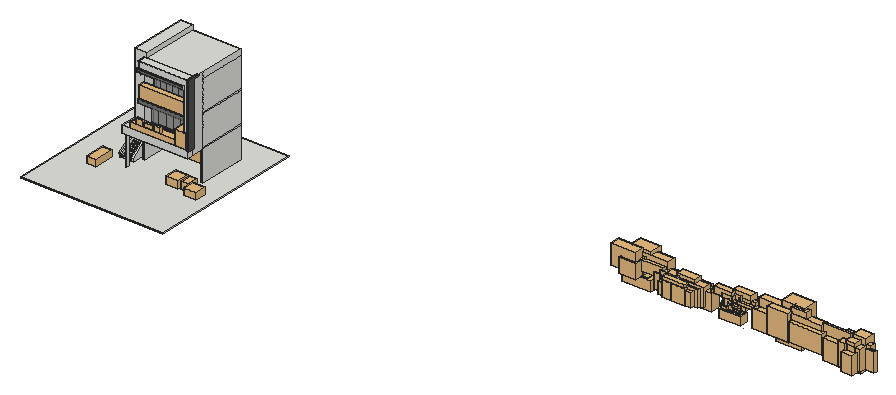
# SketchUp Ruby script. Lengths in inches.
U = 1.inch
M = Sketchup.active_model
def pt(a) = Geom::Point3d.new(a.map { |v| v * U })
def face(e, loops, mat)
  f = e.add_face(loops[0].map { |a| pt(a) })
  loops[1..].each { |l| e.add_face(l.map { |a| pt(a) }).erase! }
  f.material = f.back_material = mat if mat
  f
end
# faces: each face lists its corners as indices into pts; further lists are holes
def faces(e, pts, list, mat = nil) = list.each { |f| face(e, (f[0].is_a?(Array) ? f : [f]).map { |l| l.map { |i| pts[i] } }, mat) }
# xy, xz, yz: faces in a plane at the given z, y or x. An outline is a flat list of corners, or four numbers for a rectangle; further outlines are holes
def ring(l) = l.size == 4 ? [[l[0], l[1]], [l[2], l[1]], [l[2], l[3]], [l[0], l[3]]] : l.each_slice(2).to_a
def flat(e, list, mat, &to3) = list.each { |f| face(e, (f[0].is_a?(Array) ? f : [f]).map { |l| ring(l).map { |u, v| to3.(u, v) } }, mat) }
def xy(e, z, list, mat = nil) = flat(e, list, mat) { |x, y| [x, y, z] }
def xz(e, y, list, mat = nil) = flat(e, list, mat) { |x, z| [x, y, z] }
def yz(e, x, list, mat = nil) = flat(e, list, mat) { |y, z| [x, y, z] }
def lines(e, pts, list) = list.each { |a, b| e.add_line(pt(pts[a]), pt(pts[b])) }
# prism: a flat outline (further loops are holes) pulled along v
def prism(e, loops, v, mat = nil)
  f = face(e, loops, mat); d = Geom::Vector3d.new(v.map { |x| x * U })
  f.pushpull(f.normal.samedirection?(d) ? d.length : -d.length)
end
def box(e, o, s, mat = nil) = prism(e, [[o, [o[0] + s[0], o[1], o[2]], [o[0] + s[0], o[1] + s[1], o[2]], [o[0], o[1] + s[1], o[2]]]], [0, 0, s[2]], mat)
def at(x, y, z, deg = 0) = Geom::Transformation.translation(pt([x, y, z])) * Geom::Transformation.rotation(ORIGIN, Z_AXIS, deg.degrees)
def axes(o, x, y, z) = Geom::Transformation.new([*x, 0, *y, 0, *z, 0, *pt(o).to_a, 1])
def part(name) = M.definitions.add(name)
# library, detail: a bought-in or finely detailed component or shape, given as its bounding box
def library(name, o, s) = part(name).tap { |d| box(d.entities, o, s) }
def detail(e, o, s) = box(e.add_group.entities, o, s)
def put(e, d, t, mat = nil) = e.add_instance(d, t).tap { |i| i.material = mat if mat }
def group(e, t, mat = nil) = e.add_group.tap { |g| g.transformation = t; g.material = mat if mat }.entities
root = M.entities
M.materials.add("BANANA_BIG_STVOL_1").color = [93, 83, 53]
M.materials.add("POT_TEXTURE_1").color = [172, 172, 172]
M.materials.add("POT_TEXTURE_2").color = [160, 154, 144]
M.materials.add("[0135_DarkGray]").color = [81, 81, 81]
M.materials.add("[Color D06]").color = [204, 153, 0]
M.materials.add("[Metal Seamed]").color = [118, 119, 115]
M.materials.add("[Translucent Glass Sky Reflection]").color = [126, 138, 183]
M.materials["[Translucent Glass Sky Reflection]"].alpha = 0.52
M.materials.add("[Translucent_Glass_Gray]").color = [128, 128, 128]
M.materials["[Translucent_Glass_Gray]"].alpha = 0.5
M.materials.add("[Wood Square Tile 01]").color = [164, 91, 44]
M.materials.add("soil1").color = [68, 55, 47]
M.materials.add("white_concrete_pot1").color = [212, 211, 204]
M.materials.add("wood_1").color = [140, 119, 94]
c1 = library("sliding+glass+door+with+curtain",[16.58,6.29,0],[12.8,171.26,109.24])
c2 = part("Group\#3")
prism(c2.entities,[[[0,0,-94.49],[0,0,23.62],[-248.03,0,23.62],[-248.03,0,0],[-15.75,0,0],[-15.75,0,-94.49]]],[0,3.9375,0])
c3 = part("Group\#6")
prism(c3.entities,[[[0,0,1.97],[0,0,0],[0,1.97,0],[0,1.97,1.97],[0,1.88,2.12],[0,1.8,2.27],[0,1.73,2.42],[0,1.66,2.58],[0,1.61,2.75],[0,1.56,2.91],[0,1.52,3.08],[0,1.49,3.25],[0,1.47,3.42],[0,1.45,3.59],[0,1.45,3.76],[0,1.45,3.9375],[0,1.22,3.9375],[0,1.22,2.76],[0,0.75,2.76],[0,0.75,3.9375],[0,0.5,3.9375],[0,0.51,3.77],[0,0.5,3.59],[0,0.49,3.42],[0,0.47,3.25],[0,0.44,3.08],[0,0.4,2.91],[0,0.36,2.75],[0,0.3,2.59],[0,0.24,2.43],[0,0.17,2.27],[0,0.09,2.12]]],[-31.5,0,0])
c4 = part("Group\#8")
box(c4.entities,[-31.5,0.04,0],[31.5,0.39,88.98])
c5 = part("Group\#12")
put(c5.entities,c3,at(31.5,0,0))
put(c5.entities,c3,axes([31.5,0,94.49],[1,0,0],[0,1,0],[0,0,-1]))
put(c5.entities,c4,at(31.5,0.75,2.76),"[Translucent_Glass_Gray]")
c6 = part("Group\#9")
g1 = group(c6.entities,at(31.5,0,0))
prism(g1,[[[0,0,1.97],[0,0,0],[0,1.97,0],[0,1.97,1.97],[0,1.88,2.12],[0,1.8,2.27],[0,1.73,2.42],[0,1.66,2.58],[0,1.61,2.75],[0,1.56,2.91],[0,1.52,3.08],[0,1.49,3.25],[0,1.47,3.42],[0,1.45,3.59],[0,1.45,3.76],[0,1.45,3.9375],[0,1.22,3.9375],[0,1.22,2.76],[0,0.75,2.76],[0,0.75,3.9375],[0,0.5,3.9375],[0,0.51,3.77],[0,0.5,3.59],[0,0.49,3.42],[0,0.47,3.25],[0,0.44,3.08],[0,0.4,2.91],[0,0.36,2.75],[0,0.3,2.59],[0,0.24,2.43],[0,0.17,2.27],[0,0.09,2.12]]],[-126.8,0,0])
g2 = group(c6.entities,at(31.5,0,94.49))
prism(g2,[[[0,0,-1.97],[0,0,0],[0,1.97,0],[0,1.97,-1.97],[0,1.88,-2.12],[0,1.8,-2.27],[0,1.73,-2.42],[0,1.66,-2.58],[0,1.61,-2.75],[0,1.56,-2.91],[0,1.52,-3.08],[0,1.49,-3.25],[0,1.47,-3.42],[0,1.45,-3.59],[0,1.45,-3.76],[0,1.45,-3.9375],[0,1.22,-3.9375],[0,1.22,-2.76],[0,0.75,-2.76],[0,0.75,-3.9375],[0,0.5,-3.9375],[0,0.51,-3.77],[0,0.5,-3.59],[0,0.49,-3.42],[0,0.47,-3.25],[0,0.44,-3.08],[0,0.4,-2.91],[0,0.36,-2.75],[0,0.3,-2.59],[0,0.24,-2.43],[0,0.17,-2.27],[0,0.09,-2.12]]],[-126.8,0,0])
put(c6.entities,c4,axes([31.5,0.75,2.76],[1.00645,0,0],[0,1,0],[0,0,1]),"[Translucent_Glass_Gray]")
g3 = group(c6.entities,at(-0.2,0.75,1.69),"[Translucent_Glass_Gray]")
box(g3,[-31.7,0.04,0],[31.7,0.39,88.98])
put(c6.entities,c4,axes([-63.6,0.75,1.69],[1.00645,0,0],[0,1,0],[0,0,1]),"[Translucent_Glass_Gray]")
put(c6.entities,c4,axes([-31.9,0.75,2.76],[1.00645,0,0],[0,1,0],[0,0,1]),"[Translucent_Glass_Gray]")
c7 = library("Group\#15",[0,0,0],[5.75,8.11,23.98])
c8 = part("Glass+door\#1")
g4 = group(c8.entities,at(51.03,8.46,0))
box(g4,[0,0,0],[15.75,15.75,118.11])
g5 = group(c8.entities,at(314.81,8.46,0))
box(g5,[0,-47.24,0],[31.93,62.99,118.11])
put(c8.entities,c2,at(314.81,8.46,94.49))
put(c8.entities,c5,axes([262.72,8.46,0],[1.1514,0,0],[0,1,0],[0,0,1]))
g6 = group(c8.entities,at(226.22,8.46,0))
put(g6,c3,axes([36.26,0,0],[1.1514,0,0],[0,1,0],[0,0,1]))
put(g6,c3,axes([36.26,0,94.49],[1.1514,0,0],[0,1,0],[0,0,-1]))
put(g6,c4,axes([36.26,0.75,2.76],[1.1514,0,0],[0,1,0],[0,0,1]),"[Translucent_Glass_Gray]")
put(c8.entities,c6,axes([186.38,8.46,0],[1.25503,0,0],[0,1,0],[0,0,1]))
put(c8.entities,c7,at(259.49,5.39,34.67))
c9 = library("Glass+Railing+2",[-45.31,-3.1875,0],[166.37,85.24,47.24])
c10 = library("Beach+chair+Spa+DEDON",[0,0,0],[79.35,36.08,25.98])
c11 = library("Folding deck chair",[-1.04,-0.49,0],[50.41,43.41,27.36])
c12 = library("Folding deck chair \#1",[-1.0625,-0.61,0],[27.15,43.98,27.36])
c13 = library("Folding deck chair \#2",[-0.98,-1.27,0],[47,50.11,27.36])
c14 = library("Sliding Single Door",[0,-2.3125,0],[59.06,6.98,82.68])
c15 = library("Group\#35",[-312.76,2118.02,370.79],[80.37,61.43,57.53])
c16 = library("Group\#56",[-146.29,2044.53,349.125],[81,53.32,37.9])
c17 = library("Group\#99",[-236.03,2064.57,238.29],[378.97,266.89,1422.96])
c18 = library("Group\#44",[-392.38,2142.99,345.23],[79.77,60.6,39.05])
c19 = library("Group\#71",[-390.04,2074.71,363.78],[77.3,84.83,61.55])
c20 = library("Group\#48",[-389.63,2051.04,359.41],[56.81,81.38,37.86])
c21 = library("Group\#52",[-362.86,1963.26,351.01],[55.56,80.44,37.9])
c22 = library("Group\#55",[-200.52,1998.86,370.22],[77.15,68.38,35.39])
c23 = library("Group\#67",[-480.58,1843.32,11.96],[467.85,466.24,378.92])
c24 = library("Group\#45",[-433.57,2042.61,369.7],[71.79,72.8,37.85])
c25 = library("Group\#42",[-148.5,2084.1,354.63],[73.89,71.73,39.48])
c26 = library("Group\#81",[-372.4375,2154.5,374],[76.125,67.08,39.0625])
c27 = library("Group\#82",[-275.5,2156.34,352.11],[71.39,73.27,44.69])
c28 = library("Group\#61",[-143.56,2061.14,371.42],[79.79,63.19,51.3])
c29 = library("Group\#70",[-363.89,1895.22,354.63],[76.92,66.54,39.48])
c30 = library("Group\#63",[-145.08,2015.32,369.99],[82.29,54.05,37.9])
c31 = library("Group\#79",[-315.77,2202.04,371],[80.74,54.44,37.85])
c32 = library("Group\#72",[-419.21,1941.11,355.02],[73.1,71.21,39.06])
c33 = library("Group\#75",[-229.79,1894.04,351.01],[79.82,63.55,37.9])
c34 = library("Group\#86",[-234.26,2180.97,367.05],[50.63,74.65,43.95])
c35 = library("Group\#88",[-904.81,1865.01,156.3],[624.43,217.34,1227.7])
c36 = library("Group\#89",[-312.51,1611.52,263.78],[120.52,408.52,1275.1])
c37 = library("Group\#90",[-571.16,1736.08,232.33],[294.08,306.57,1438.75])
c38 = library("Group\#92",[-273.21,1593.22,47.51],[374.54,419.07,1416.6])
c39 = library("Group\#39",[-202.35,1900.5,372.29],[58.53,80.11,50.06])
c40 = library("Group\#47",[-432.01,1984.38,372.6875],[64.1,75.95,39.0625])
c41 = library("Group\#60",[-310.7,1952.62,354.63],[79.53,58.52,39.48])
c42 = library("Group\#46",[-374.28,1979.7,369.99],[51.81,82.66,37.9])
c43 = library("Group\#77",[-397.18,1916.74,372.44],[70.02,74.57,49.25])
c44 = library("Group\#84",[-236.3,2186.8,344.47],[79.26,62.91,39.06])
c45 = library("Group\#38",[-161.07,2117.49,373.61],[81.25,53.73,39.48])
c46 = library("Group\#87",[-431.9,1883.46,368.72],[373.65,376.39,18.61])
c47 = library("Group\#59",[-340.96,1970.4,361.28],[81.22,51.59,61.62])
c48 = library("Group\#65",[-272.7,1884.51,369.99],[80.39,55.87,37.9])
c49 = library("Group\#54",[-330.83,2117.69,370.2],[61.83,80.2,35.55])
c50 = library("Group\#85",[-366.3125,2177.8,359.41],[79.9,61.23,37.86])
c51 = library("Group\#51",[-435.875,2067.96,347.82],[58.32,80.53,38.29])
c52 = library("Group\#83",[-183.79,2161.45,371.25],[72.43,70.21,54.35])
c53 = library("Group\#91",[-208.23,2037.18,75.37],[621.09,225.61,1251.82])
c54 = library("Group\#94",[-675.58,1862.05,152.55],[378.81,196.01,1743.84])
c55 = library("Group\#95",[-257.06,2048.08,160.05],[394.6,177.93,1743.83])
c56 = library("Group\#96",[-344.84,1500.61,160.55],[176.35,551.19,1921.45])
c57 = library("Group\#97",[-231.77,1913.24,119.96],[448.93,143.84,1582.05])
c58 = library("Group\#98",[-616.67,2098.6,178.29],[331.19,111.16,1177.92])
c59 = library("Group\#93",[-527.15,2088.47,150.96],[267.01,328.12,1599.25])
c60 = library("Group\#100",[-792.12,2067.32,152.13],[549.56,259.52,1931.8])
c61 = library("Group\#101",[-281.17,2118.67,243.77],[133.23,408.71,1313.3])
c62 = part("Potted foliage plant")
g7 = group(c62.entities,at(904.81,-1500.61,-11.96),"white_concrete_pot1")
detail(g7,[-222.14,2117.95,372.07],[61.87,75.41,50.35])
put(c62.entities,c15,at(904.81,-1500.61,-11.96),"white_concrete_pot1")
g8 = group(c62.entities,at(904.81,-1500.61,-11.96),"white_concrete_pot1")
detail(g8,[-313.93,1881.02,351.21],[70.15,73.18,37.2])
g9 = group(c62.entities,at(904.81,-1500.61,-11.96),"white_concrete_pot1")
detail(g9,[-209.1,1970.26,378.89],[50.57,81.04,37.2])
put(c62.entities,c16,at(904.81,-1500.61,-11.96),"white_concrete_pot1")
put(c62.entities,c17,at(904.81,-1500.61,-11.96))
put(c62.entities,c18,at(904.81,-1500.61,-11.96),"white_concrete_pot1")
put(c62.entities,c19,at(904.81,-1500.61,-11.96),"white_concrete_pot1")
put(c62.entities,c20,at(904.81,-1500.61,-11.96),"white_concrete_pot1")
put(c62.entities,c21,at(904.81,-1500.61,-11.96),"white_concrete_pot1")
g10 = group(c62.entities,at(904.81,-1500.61,-11.96),"white_concrete_pot1")
detail(g10,[-129.49,1972.75,359.91],[55.59,80.76,37.2])
put(c62.entities,c22,at(904.81,-1500.61,-11.96),"white_concrete_pot1")
g11 = group(c62.entities,at(904.81,-1500.61,-11.96),"white_concrete_pot1")
detail(g11,[-333.13,1892.25,370.19],[61.39,79.4,37.2])
put(c62.entities,c23,at(904.81,-1500.61,-11.96),"POT_TEXTURE_1")
put(c62.entities,c24,at(904.81,-1500.61,-11.96),"white_concrete_pot1")
put(c62.entities,c25,at(904.81,-1500.61,-11.96),"white_concrete_pot1")
g12 = group(c62.entities,at(904.81,-1500.61,-11.96),"white_concrete_pot1")
detail(g12,[-270.91,2176.57,345.18],[52.11,82.01,38.29])
g13 = group(c62.entities,at(904.81,-1500.61,-11.96),"white_concrete_pot1")
detail(g13,[-195.71,2019.1875,371.11],[58.98,81.18,37.2])
g14 = group(c62.entities,at(904.81,-1500.61,-11.96),"white_concrete_pot1")
detail(g14,[-319.36,2078.81,339.18],[76.07,69.08,39.48])
put(c62.entities,c26,at(904.81,-1500.61,-11.96),"white_concrete_pot1")
put(c62.entities,c27,at(904.81,-1500.61,-11.96),"white_concrete_pot1")
g15 = group(c62.entities,at(904.81,-1500.61,-11.96),"white_concrete_pot1")
detail(g15,[-417.64,2112.53,369.82],[65.44,79.59,38.29])
put(c62.entities,c28,at(904.81,-1500.61,-11.96),"white_concrete_pot1")
put(c62.entities,c29,at(904.81,-1500.61,-11.96),"white_concrete_pot1")
put(c62.entities,c30,at(904.81,-1500.61,-11.96),"white_concrete_pot1")
g16 = group(c62.entities,at(904.81,-1500.61,-11.96),"white_concrete_pot1")
detail(g16,[-240.6,2054.85,378.89],[71.5,72.03,37.2])
put(c62.entities,c31,at(904.81,-1500.61,-11.96),"white_concrete_pot1")
put(c62.entities,c32,at(904.81,-1500.61,-11.96),"white_concrete_pot1")
put(c62.entities,c33,at(904.81,-1500.61,-11.96),"white_concrete_pot1")
g17 = group(c62.entities,at(904.81,-1500.61,-11.96),"white_concrete_pot1")
detail(g17,[-249.82,2117.53,359.91],[58.07,81.25,37.2])
put(c62.entities,c34,at(904.81,-1500.61,-11.96),"white_concrete_pot1")
put(c62.entities,c35,at(904.81,-1500.61,-11.96))
put(c62.entities,c36,at(904.81,-1500.61,-11.96))
put(c62.entities,c37,at(904.81,-1500.61,-11.96))
put(c62.entities,c38,at(904.81,-1500.61,-11.96))
g18 = group(c62.entities,at(904.81,-1500.61,-11.96),"white_concrete_pot1")
detail(g18,[-435.4375,2027.54,350.71],[78.74,62.6,37.86])
put(c62.entities,c39,at(904.81,-1500.61,-11.96),"white_concrete_pot1")
g19 = group(c62.entities,at(904.81,-1500.61,-11.96),"white_concrete_pot1")
detail(g19,[-173.8,2126.25,354.63],[80.17,60.53,39.48])
g20 = group(c62.entities,at(904.81,-1500.61,-11.96),"white_concrete_pot1")
detail(g20,[-222.96,2066.75,359.91],[63.77,78.21,37.2])
put(c62.entities,c40,at(904.81,-1500.61,-11.96),"white_concrete_pot1")
g21 = group(c62.entities,at(904.81,-1500.61,-11.96),"white_concrete_pot1")
detail(g21,[-183.125,1913.38,330.04],[66.78,77.69,39.48])
put(c62.entities,c41,at(904.81,-1500.61,-11.96),"white_concrete_pot1")
g22 = group(c62.entities,at(904.81,-1500.61,-11.96),"white_concrete_pot1")
detail(g22,[-152,1936.85,378.89],[64.46,79.76,37.2])
g23 = group(c62.entities,at(904.81,-1500.61,-11.96),"white_concrete_pot1")
detail(g23,[-284.65,1933.22,373.64],[80.83,55.23,37.2])
put(c62.entities,c42,at(904.81,-1500.61,-11.96),"white_concrete_pot1")
g24 = group(c62.entities,at(904.81,-1500.61,-11.96),"white_concrete_pot1")
detail(g24,[-263.49,1923.54,359.91],[75.98,66.75,37.2])
put(c62.entities,c43,at(904.81,-1500.61,-11.96),"white_concrete_pot1")
g25 = group(c62.entities,at(904.81,-1500.61,-11.96),"white_concrete_pot1")
detail(g25,[-167.97,1940.97,354.63],[66.78,77.7,39.48])
put(c62.entities,c44,at(904.81,-1500.61,-11.96),"white_concrete_pot1")
g26 = group(c62.entities,at(904.81,-1500.61,-11.96),"white_concrete_pot1")
detail(g26,[-214.75,1956.59,330.04],[66.78,77.69,39.48])
put(c62.entities,c45,at(904.81,-1500.61,-11.96),"white_concrete_pot1")
put(c62.entities,c46,at(904.81,-1500.61,-11.96),"white_concrete_pot1")
put(c62.entities,c47,at(904.81,-1500.61,-11.96),"white_concrete_pot1")
g27 = group(c62.entities,at(904.81,-1500.61,-11.96),"white_concrete_pot1")
detail(g27,[-282.5625,1934.21,389.56],[81.1,59.19,35.03])
put(c62.entities,c48,at(904.81,-1500.61,-11.96),"white_concrete_pot1")
g28 = group(c62.entities,at(904.81,-1500.61,-11.96),"white_concrete_pot1")
detail(g28,[-394.5,2036.48,359.91],[79.58,64.84,37.2])
put(c62.entities,c49,at(904.81,-1500.61,-11.96),"white_concrete_pot1")
put(c62.entities,c50,at(904.81,-1500.61,-11.96),"white_concrete_pot1")
put(c62.entities,c51,at(904.81,-1500.61,-11.96),"white_concrete_pot1")
put(c62.entities,c52,at(904.81,-1500.61,-11.96),"white_concrete_pot1")
put(c62.entities,c53,at(904.81,-1500.61,-11.96))
put(c62.entities,c54,at(904.81,-1500.61,-11.96))
put(c62.entities,c55,at(904.81,-1500.61,-11.96))
put(c62.entities,c56,at(904.81,-1500.61,-11.96))
put(c62.entities,c57,at(904.81,-1500.61,-11.96))
put(c62.entities,c58,at(904.81,-1500.61,-11.96))
put(c62.entities,c59,at(904.81,-1500.61,-11.96))
put(c62.entities,c60,at(904.81,-1500.61,-11.96))
put(c62.entities,c61,at(904.81,-1500.61,-11.96))
c63 = library("Group\#109",[-662.41,217.3,320.04],[397.32,658.3,1732.06])
c64 = library("Group\#111",[-299.2,181.55,262.58],[360.65,735.71,1258.34])
c65 = library("Group\#106",[-1038.76,656.55,345.34],[733.18,460.51,2065.7])
c66 = library("Group\#104",[-445.29,890.31,329.28],[284.3,304.08,2023.29])
c67 = library("Group\#107",[-733.48,439.625,202.64],[456.28,533.12,1536.78])
c68 = library("Group\#110",[-455.56,899.32,410.78],[341.21,610.33,1581.5])
c69 = library("Group\#103",[-516.34,626.77,-4.5625],[517.73,515.95,418.98])
c70 = library("Group\#108",[-249.24,914.85,310.18],[345.55,647.95,1307.93])
c71 = library("Group\#105",[-277.97,488.68,287.26],[362.84,405.94,1768.54])
c72 = library("Group\#102",[-468.76,669.89,380.1875],[424.36,427.47,41.99])
c73 = part("Potted tropical plant")
put(c73.entities,c63,at(1038.76,-181.55,4.5625))
put(c73.entities,c64,at(1038.76,-181.55,4.5625))
put(c73.entities,c65,at(1038.76,-181.55,4.5625))
put(c73.entities,c66,at(1038.76,-181.55,4.5625))
put(c73.entities,c67,at(1038.76,-181.55,4.5625))
put(c73.entities,c68,at(1038.76,-181.55,4.5625))
put(c73.entities,c69,at(1038.76,-181.55,4.5625),"POT_TEXTURE_1")
put(c73.entities,c70,at(1038.76,-181.55,4.5625))
put(c73.entities,c71,at(1038.76,-181.55,4.5625))
put(c73.entities,c72,at(1038.76,-181.55,4.5625),"soil1")
c74 = library("Group\#115",[-246.45,-349.05,558.47],[136.91,100.49,66.1])
c75 = library("Group\#118",[-264.68,-415.73,1484.11],[304.64,209.69,227.41])
c76 = library("Group\#125",[-357.04,-394.18,1447.05],[213.62,306.36,356.95])
c77 = library("Group\#113",[-447.02,-464.95,536.35],[343.73,346.24,39.39])
c78 = library("Group\#114",[-394.9,-448.99,911.74],[90.19,96.88,85.93])
c79 = library("Group\#124",[-424,-312.27,817.53],[158.81,108.06,136.45])
c80 = library("Group\#128",[-409.02,-515.05,915.53],[69.62,77.27,65.47])
c81 = library("Group\#132",[-548.25,-262.82,1459.54],[373.26,352.35,568])
c82 = library("Group\#139",[-492.14,-508.4,-4.15],[433.72,431.71,567.03])
c83 = library("Group\#135",[-293.78,-482.77,597.9],[158.75,112.78,159.87])
c84 = library("Group\#119",[-545.09,-386.51,922.3125],[300.25,219.65,227.33])
c85 = library("Group\#137",[-292.81,-667.38,1418.14],[215.17,356.07,188.87])
c86 = library("Group\#121",[-292.14,-288.9,1281.79],[169.55,204.34,203.36])
c87 = library("Group\#126",[-568.91,-444.37,1285.4],[307.6,179.39,277.93])
c88 = library("Group\#123",[-341.93,-403.49,744.8125],[64.83,96.32,132.15])
c89 = library("Group\#112",[-258.04,-282.68,604.05],[115.53,137.01,52.63])
c90 = library("Group\#120",[-304.79,-269.16,622.65],[82.06,111.89,102.57])
c91 = library("Group\#127",[-388.93,-514.39,838.93],[89.79,77.73,82.08])
c92 = library("Group\#129",[-295.03,-516.52,742.34],[68.71,141.75,78.67])
c93 = library("Group\#136",[-422.77,-235.4,843.61],[178.54,197.77,233.54])
c94 = library("Group\#130",[-498.98,-524.4,908.45],[120.83,107.95,112.98])
c95 = library("Group\#133",[-321.08,-139.66,1308.49],[285.55,393.29,221.53])
c96 = library("Group\#131",[-278.4,-571.99,1530.91],[311.57,345.77,423.62])
c97 = library("Group\#134",[-387.74,-136.11,1470.07],[230,321.58,230.27])
c98 = library("Group\#122",[-244.55,-305.59,1009.46],[103.13,76.81,77.34])
c99 = library("Group\#138",[-385.21,-446.52,494.02],[160.93,321.12,1142.36])
c100 = library("Group\#116",[-249.18,-250.59,980.93],[152.21,116.16,134.05])
c101 = library("Group\#117",[-438.92,-265.61,702.3],[171.52,146.16,133.5])
c102 = part("Potted broadleaf plant")
p = [[568.91,667.38,4.15],[569.91,667.38,4.15],[569.91,668.38,4.15]]
lines(c102.entities,p,[[0,1],[1,2],[2,0]])
put(c102.entities,c74,at(568.91,667.38,4.15))
put(c102.entities,c75,at(568.91,667.38,4.15))
put(c102.entities,c76,at(568.91,667.38,4.15))
put(c102.entities,c77,at(568.91,667.38,4.15),"soil1")
put(c102.entities,c78,at(568.91,667.38,4.15))
put(c102.entities,c79,at(568.91,667.38,4.15))
put(c102.entities,c80,at(568.91,667.38,4.15))
put(c102.entities,c81,at(568.91,667.38,4.15))
put(c102.entities,c82,at(568.91,667.38,4.15),"POT_TEXTURE_2")
put(c102.entities,c83,at(568.91,667.38,4.15))
put(c102.entities,c84,at(568.91,667.38,4.15))
put(c102.entities,c85,at(568.91,667.38,4.15))
put(c102.entities,c86,at(568.91,667.38,4.15))
put(c102.entities,c87,at(568.91,667.38,4.15))
put(c102.entities,c88,at(568.91,667.38,4.15))
put(c102.entities,c89,at(568.91,667.38,4.15))
put(c102.entities,c90,at(568.91,667.38,4.15))
put(c102.entities,c91,at(568.91,667.38,4.15))
put(c102.entities,c92,at(568.91,667.38,4.15))
put(c102.entities,c93,at(568.91,667.38,4.15))
put(c102.entities,c94,at(568.91,667.38,4.15))
put(c102.entities,c95,at(568.91,667.38,4.15))
put(c102.entities,c96,at(568.91,667.38,4.15))
put(c102.entities,c97,at(568.91,667.38,4.15))
put(c102.entities,c98,at(568.91,667.38,4.15))
put(c102.entities,c99,at(568.91,667.38,4.15),"wood_1")
put(c102.entities,c100,at(568.91,667.38,4.15))
put(c102.entities,c101,at(568.91,667.38,4.15))
c103 = library("Group\#147",[-640.625,-1318.37,287.11],[396.64,314.81,689.96])
c104 = library("Group\#142",[-513.94,-1201.2,195.17],[480.66,557.42,1160.08])
c105 = library("Group\#144",[-208.03,-1336.63,286.21],[381.72,484.79,1145.39])
c106 = library("Group\#150",[-619.83,-1636.3,288.9],[316.15,456.61,1171.28])
c107 = library("Group\#151",[-738.91,-1210.08,301],[426.4,388.88,1000.79])
c108 = library("Group\#153",[-208.33,-1511.76,297.04],[508.2,421.96,1258.76])
c109 = library("Group\#143",[-545.36,-1775.03,287.125],[412.21,432,920.68])
c110 = library("Group\#148",[-750.24,-1478.51,301.56],[423.84,451.05,998.69])
c111 = library("Group\#146",[-245.33,-1174.2,301.22],[356.02,306.31,608.34])
c112 = library("Group\#141",[-487.23,-1483.58,-4.71],[450.86,446.99,418.38])
c113 = library("Group\#155",[-445.7,-1606.55,154.18],[255.44,283.57,849.28])
c114 = library("Group\#156",[-390.1,-1177.12,195.59],[220.93,265.44,790.12])
c115 = library("Group\#158",[-480.32,-1333.42,295.8],[424.49,356.06,1482.77])
c116 = library("Group\#159",[-378.01,-1245.98,305.66],[422.15,474.55,1267.42])
c117 = library("Group\#145",[-163.65,-1622.09,292.29],[406.18,374.8,780.12])
c118 = library("Group\#154",[-384.8,-1640.99,300.61],[422.68,348.03,1297.96])
c119 = library("Group\#140",[-429.18,-1441.17,362.05],[345.84,348.28,45.35])
c120 = library("Group\#157",[-208.0625,-1498.77,286.27],[547.26,435.76,1075.6])
c121 = library("Group\#152",[-172.82,-1329.68,294.68],[502.85,397.72,955.79])
c122 = library("Group\#149",[-426.76,-1753.59,287.48],[479.67,412.35,1049.19])
c123 = part("Potted palm")
put(c123.entities,c103,at(750.24,1775.03,4.71))
put(c123.entities,c104,at(750.24,1775.03,4.71))
put(c123.entities,c105,at(750.24,1775.03,4.71))
put(c123.entities,c106,at(750.24,1775.03,4.71))
put(c123.entities,c107,at(750.24,1775.03,4.71))
put(c123.entities,c108,at(750.24,1775.03,4.71))
put(c123.entities,c109,at(750.24,1775.03,4.71))
put(c123.entities,c110,at(750.24,1775.03,4.71))
put(c123.entities,c111,at(750.24,1775.03,4.71))
put(c123.entities,c112,at(750.24,1775.03,4.71),"POT_TEXTURE_1")
put(c123.entities,c113,at(750.24,1775.03,4.71))
put(c123.entities,c114,at(750.24,1775.03,4.71))
put(c123.entities,c115,at(750.24,1775.03,4.71))
put(c123.entities,c116,at(750.24,1775.03,4.71))
put(c123.entities,c117,at(750.24,1775.03,4.71))
put(c123.entities,c118,at(750.24,1775.03,4.71))
put(c123.entities,c119,at(750.24,1775.03,4.71),"soil1")
put(c123.entities,c120,at(750.24,1775.03,4.71))
put(c123.entities,c121,at(750.24,1775.03,4.71))
put(c123.entities,c122,at(750.24,1775.03,4.71))
c124 = library("Group\#160",[-480.3,-2300.47,677.45],[398.14,398.43,28.25])
c125 = library("Group\#161",[-336.38,-2175.79,614.41],[133.99,147.1,560.64])
c126 = library("Group\#162",[-311.45,-2362.85,663.67],[597.01,322.07,1007.38])
c127 = library("Group\#163",[-330.26,-2159.14,612.04],[116.66,119.22,673.97])
c128 = library("Group\#164",[-667.53,-2111.4375,1071.74],[420.02,555.28,968.03])
c129 = library("Group\#165",[-328.97,-2115.58,1156.29],[117.86,119.42,695.38])
c130 = library("Group\#166",[-943.22,-2312.1875,967.59],[670.63,402.45,1245.73])
c131 = library("Group\#168",[-343.93,-2076.42,1024.91],[285.05,475.82,708.21])
c132 = library("Group\#167",[-568.09,-2386.9,-3.76],[573.62,569.18,700.28])
c133 = library("Group\#169",[-550.09,-2664.39,1031.96],[371.42,533.86,798])
c134 = library("Group\#170",[-308.37,-2556.11,869.35],[483.58,483.6,1385.8])
c135 = part("Potted tropical plant \#1")
put(c135.entities,c124,at(943.22,2664.39,3.76),"soil1")
put(c135.entities,c125,at(943.22,2664.39,3.76),"BANANA_BIG_STVOL_1")
put(c135.entities,c126,at(943.22,2664.39,3.76))
put(c135.entities,c127,at(943.22,2664.39,3.76),"BANANA_BIG_STVOL_1")
put(c135.entities,c128,at(943.22,2664.39,3.76))
put(c135.entities,c129,at(943.22,2664.39,3.76))
put(c135.entities,c130,at(943.22,2664.39,3.76))
put(c135.entities,c131,at(943.22,2664.39,3.76))
put(c135.entities,c132,at(943.22,2664.39,3.76),"POT_TEXTURE_2")
put(c135.entities,c133,at(943.22,2664.39,3.76))
put(c135.entities,c134,at(943.22,2664.39,3.76))
c136 = part("plants")
put(c136.entities,c62,at(-904.81,1500.61,11.96))
put(c136.entities,c73,at(-1038.76,181.55,-4.5625))
put(c136.entities,c102,at(-568.91,-667.38,-4.15))
put(c136.entities,c123,at(-750.24,-1775.03,-4.71))
put(c136.entities,c135,at(-943.22,-2664.39,-3.76))
c137 = library("Potted peace lily",[-1.15,-1.29,0],[7.65,7.78,5.89])
c138 = library("trol",[-1.07,-0.37,0],[9.56,15.9,13.04])
c139 = library("KentiaPalm",[-22.86,-14.31,0],[47.49,43.96,59.125])
xy(root,0,[[0,0,573.375,632.3125]])
xy(root,2,[[[0,0,573.375,632.3125],[169.29,298.14,205.29,308.14]],[169.29,298.14,205.29,308.14]])
xy(root,8,[[169.29,298.14,205.29,308.14],[169.29,308.14,205.29,318.14]])
xy(root,14,[[169.29,308.14,205.29,318.14],[169.29,318.14,205.29,328.14]])
xy(root,20,[[169.29,318.14,205.29,328.14],[169.29,328.14,205.29,338.14]])
xy(root,26,[[169.29,328.14,205.29,338.14],[169.29,338.14,205.29,348.14]])
xy(root,32,[[169.29,338.14,205.29,348.14],[169.29,348.14,205.29,358.14]])
xy(root,38,[[169.29,348.14,205.29,358.14],[169.29,358.14,205.29,368.14]])
xy(root,44,[[169.29,358.14,205.29,368.14],[169.29,368.14,205.29,378.14]])
xy(root,50,[[169.29,368.14,205.29,378.14],[169.29,378.14,205.29,388.14]])
xy(root,56,[[169.29,378.14,205.29,388.14],[169.29,388.14,205.29,398.14]])
xy(root,62,[[169.29,388.14,205.29,398.14],[169.29,398.14,205.29,408.14],[166.85,408.14,216.31,521.35]])
xy(root,68,[[169.29,398.14,205.29,408.14]])
xy(root,75.9375,[[166.85,408.14,216.31,521.35]])
xy(root,149.1875,[[468.97,250.96,476.78,273.71]])
xy(root,401.1875,[[468.97,273.71,476.78,299.77]])
xy(root,407.32,[[468.97,250.96,476.78,299.77]],"[0135_DarkGray]")
xz(root,0,[[0,0,573.375,2]])
xz(root,250.96,[[468.97,149.1875,476.78,407.32]],"[0135_DarkGray]")
xz(root,273.71,[[468.97,149.1875,476.78,401.1875]])
xz(root,298.14,[[169.29,2,205.29,8]])
xz(root,299.77,[[468.97,401.1875,476.78,407.32]])
xz(root,308.14,[[169.29,2,205.29,8],[169.29,8,205.29,14]])
xz(root,318.14,[[169.29,8,205.29,14],[169.29,14,205.29,20]])
xz(root,328.14,[[169.29,14,205.29,20],[169.29,20,205.29,26]])
xz(root,338.14,[[169.29,20,205.29,26],[169.29,26,205.29,32]])
xz(root,348.14,[[169.29,26,205.29,32],[169.29,32,205.29,38]])
xz(root,358.14,[[169.29,32,205.29,38],[169.29,38,205.29,44]])
xz(root,368.14,[[169.29,38,205.29,44],[169.29,44,205.29,50]])
xz(root,378.14,[[169.29,44,205.29,50],[169.29,50,205.29,56]])
xz(root,388.14,[[169.29,50,205.29,56],[169.29,56,205.29,62]])
xz(root,398.14,[[169.29,56,205.29,62],[169.29,62,205.29,68]])
xz(root,408.14,[[166.85,62,169.29,68],[169.29,62,205.29,68],[205.29,62,216.31,75.9375],[166.85,68,205.29,75.9375]])
xz(root,521.35,[[166.85,62,216.31,75.9375]])
xz(root,632.3125,[[0,0,573.375,2]])
yz(root,0,[[0,0,632.3125,2]])
yz(root,166.85,[[408.14,62,521.35,75.9375]])
yz(root,169.29,[[298.14,2,308.14,8],[308.14,8,318.14,14],[318.14,14,328.14,20],[328.14,20,338.14,26],[338.14,26,348.14,32],
  [348.14,32,358.14,38],[358.14,38,368.14,44],[368.14,44,378.14,50],[378.14,50,388.14,56],[388.14,56,398.14,62],
  [398.14,62,408.14,68]])
yz(root,205.29,[[298.14,2,308.14,8],[308.14,8,318.14,14],[318.14,14,328.14,20],[328.14,20,338.14,26],[338.14,26,348.14,32],
  [348.14,32,358.14,38],[358.14,38,368.14,44],[368.14,44,378.14,50],[378.14,50,388.14,56],[388.14,56,398.14,62],
  [398.14,62,408.14,68]])
yz(root,216.31,[[408.14,62,521.35,75.9375]])
yz(root,468.97,[[250.96,149.1875,250.96,407.32,299.77,407.32,299.77,401.1875,273.71,401.1875,273.71,149.1875]],"[0135_DarkGray]")
yz(root,476.78,[[250.96,149.1875,273.71,149.1875,273.71,401.1875,299.77,401.1875,299.77,407.32,250.96,407.32]],"[0135_DarkGray]")
yz(root,573.375,[[0,0,632.3125,2]])
p = [[317.17,207.8,390.65],[317.17,207.8,389.65],[377.32,477.07,149.5625],[377.32,477.07,147.95],[205.29,408.14,62],[205.29,408.14,2]]
lines(root,p,[[0,1],[2,3],[4,5]])
put(root,c1,axes([232.23,450.15,2],[0.01047,-0.99995,0],[1.26553,0.01325,0],[0,0,1.10135]),"[Translucent Glass Sky Reflection]")
put(root,c8,axes([240.24,327.43,263.9375],[0.59107,0,0],[0,0.1095,0],[0,0,0.95054]))
put(root,c9,axes([315.57,264.4375,263.9375],[1.11,0,0],[0,0.3,0],[0,0,1]))
put(root,c9,axes([297.34,259.1,141.6875],[1.3986,0,0],[0,0.36,0],[0,0,0.56832]))
put(root,c10,at(143.4375,199.4,2,90))
put(root,c11,at(474.46,229.61,2.28))
put(root,c12,at(443.21,256.29,2.28))
put(root,c13,at(385.04,252.19,2))
put(root,c14,at(224.83,427.3,262.64,-90))
put(root,c14,at(224.29,440.18,109.4,-90))
put(root,c136,axes([2370.55,671.96,-4.44],[0,-0.07665,0],[0.2044,0,0],[0,0,0.0574]))
put(root,c137,axes([258.5625,269.1875,149.5625],[3.54384,0,0],[0,-1,0],[0,0,6.7276]))
put(root,c138,axes([285.22,273.63,149.5625],[0,-1,0],[2.28,0,0],[0,0,2.5]))
put(root,c139,at(437.01,271.38,149.5625))
put(root,c137,axes([328.8125,269.1875,149.5625],[3.54384,0,0],[0,-1,0],[0,0,6.7276]))
put(root,c5,axes([414.96,323.28,149.5625],[0.8495,0,0],[0,0.1991,0],[0,0,0.89]))
g29 = group(root,at(388.04,323.28,149.5625))
put(g29,c3,axes([26.76,0,0],[0.8495,0,0],[0,0.1991,0],[0,0,0.89]))
put(g29,c3,axes([26.76,0,84.09],[0.8495,0,0],[0,0.1991,0],[0,0,-0.89]))
put(g29,c4,axes([26.76,0.15,2.45],[0.8495,0,0],[0,0.1991,0],[0,0,0.89]),"[Translucent_Glass_Gray]")
put(root,c6,axes([358.64,323.28,149.5625],[0.92596,0,0],[0,0.1991,0],[0,0,0.89]))
put(root,c7,axes([412.58,322.67,180.42],[0.7378,0,0],[0,0.1991,0],[0,0,0.89]))
g30 = group(root,at(453.4,323.28,149.5625))
p = [[0,3.14,0],[0,3.14,105.12]]
lines(g30,p,[[0,1]])
put(root,c2,axes([453.4,323.28,233.66],[0.7378,0,0],[0,0.1991,0],[0,0,0.89]))
g31 = group(root,at(228.97,277.52,2))
g32 = group(g31,at(-22.875,-23.625,0))
xy(g32,0,[[9.8125,5.51,16.5,15.33],[22.875,76.1875,22.875,266.4375,262.875,266.4375,262.875,76.1875,257.41,76.1875,257.41,180,30.48,180,30.48,76.1875]])
xy(g32,120.3125,[[[0,0,0,83.39,22.875,83.39,22.875,76.1875,243.1875,76.1875,243.1875,23.625,262.875,23.625,262.875,0],[9.8125,5.51,16.5,15.33]],[9.8125,5.51,16.5,15.33],[243.1875,23.625,262.875,76.1875],[30.48,76.1875,257.41,180]])
xy(g32,147.5625,[[0,0,262.875,0,262.875,5.75,243.1875,5.75,243.1875,76.1875,64.31,76.1875,64.31,34.5625,22.875,34.5625,22.875,83.39,0,83.39],[243.1875,5.75,262.875,23.625],[22.875,34.5625,64.31,76.1875]])
xy(g32,246.3125,[[243.1875,5.75,243.8125,76.1875],[59.18,23.625,64.31,34.5625]])
xy(g32,246.3125,[[59.18,5.75,59.18,23.625,64.31,23.625,64.31,76.1875,243.1875,76.1875,243.1875,5.75]],"[Color D06]")
xy(g32,261.9375,[[59.18,5.75,243.8125,5.75,243.8125,76.1875,64.31,76.1875,64.31,34.5625,59.18,34.5625]],"[Metal Seamed]")
xy(g32,359.5,[[56.31,1.375,56.31,34.5625,64.31,34.5625,64.31,76.1875,243.8125,76.1875,243.8125,1.375]],"[Wood Square Tile 01]")
xy(g32,360,[[56.31,1.375,243.8125,2.125],[56.31,2.125,56.93,34.5625]])
xy(g32,371.8125,[[56.56,1,243.8125,2.125],[56.56,2.125,56.93,34.5625]])
xy(g32,372.3125,[[61.81,5.75,243.8125,5.75,243.8125,76.1875,64.31,76.1875,64.31,34.5625,61.81,34.5625]])
xy(g32,372.3125,[[56.56,1,243.8125,1,243.8125,5.75,61.81,5.75,61.81,34.5625,56.56,34.5625]],"[Metal Seamed]")
xy(g32,397.9375,[[60.43,5.0625,262.875,5.75]])
xy(g32,398.1875,[[60.43,5.75,61.81,34.5625]])
xy(g32,399.1875,[[60.43,5.0625,262.875,34.5625],[70.18,34.5625,262.875,266.4375]])
xy(g32,418.25,[[22.875,34.5625,70.18,266.4375]])
xz(g32,0,[[0,120.3125,262.875,147.5625]])
xz(g32,1,[[56.56,371.8125,243.8125,372.3125]],"[Metal Seamed]")
xz(g32,1.375,[[56.31,359.5,243.8125,360]],"[Metal Seamed]")
xz(g32,2.125,[[56.93,360,243.8125,371.8125]],"[Metal Seamed]")
xz(g32,5.0625,[[60.43,397.9375,262.875,399.1875]])
xz(g32,5.51,[[9.8125,0,16.5,120.3125]])
xz(g32,5.75,[[243.1875,147.5625,262.875,147.5625,262.875,397.9375,61.81,397.9375,61.81,372.3125,243.8125,372.3125,243.8125,246.3125,243.1875,246.3125],[60.43,397.9375,61.81,398.1875]])
xz(g32,5.75,[[59.18,246.3125,243.8125,261.9375]],"[Metal Seamed]")
xz(g32,15.33,[[9.8125,0,16.5,120.3125]])
xz(g32,23.625,[[243.1875,120.3125,262.875,147.5625]])
xz(g32,34.5625,[[22.875,147.5625,64.31,147.5625,64.31,246.3125,59.18,246.3125,59.18,261.9375,64.31,261.9375,64.31,359.5,56.31,359.5,56.31,360,56.93,360,56.93,371.8125,56.56,371.8125,56.56,372.3125,61.81,372.3125,61.81,398.1875,60.43,398.1875,60.43,399.1875,70.18,399.1875,70.18,418.25,22.875,418.25],[56.31,359.5,64.31,359.5,64.31,372.3125,56.56,372.3125,56.56,371.8125,56.93,371.8125,56.93,360,56.31,360]])
xz(g32,76.1875,[[22.875,0,30.48,120.3125],[257.41,0,262.875,120.3125],[243.1875,120.3125,262.875,126.3125],[22.875,126.3125,243.1875,147.5625],[243.1875,126.3125,262.875,126.3125,262.875,360.875,243.8125,360.875,243.8125,246.3125,243.1875,246.3125],
  [64.31,147.5625,243.1875,246.3125],[64.31,246.3125,243.8125,261.9375],[64.31,261.9375,243.8125,359.5],[64.31,359.5,243.8125,372.3125],[243.8125,360.875,262.875,369.1875],
  [243.8125,369.1875,262.875,372.3125]])
xz(g32,83.39,[[0,120.3125,22.875,147.5625]])
xz(g32,180,[[30.48,0,257.41,120.3125]])
xz(g32,266.4375,[[22.875,0,22.875,418.25,70.18,418.25,70.18,399.1875,262.875,399.1875,262.875,0]])
yz(g32,0,[[0,120.3125,83.39,147.5625]])
yz(g32,9.8125,[[5.51,0,15.33,120.3125]])
yz(g32,16.5,[[5.51,0,15.33,120.3125]])
yz(g32,22.875,[[76.1875,0,76.1875,120.3125,83.39,120.3125,83.39,147.5625,34.5625,147.5625,34.5625,418.25,266.4375,418.25,266.4375,0],[76.1875,126.3125,83.39,147.5625]])
yz(g32,30.48,[[76.1875,0,180,120.3125]])
yz(g32,56.31,[[1.375,359.5,34.5625,360]])
yz(g32,56.56,[[1,371.8125,34.5625,372.3125]])
yz(g32,56.93,[[2.125,360,34.5625,371.8125]],"[Metal Seamed]")
yz(g32,59.18,[[5.75,246.3125,34.5625,261.9375]],"[Metal Seamed]")
yz(g32,60.43,[[5.0625,397.9375,5.0625,399.1875,34.5625,399.1875,34.5625,398.1875,5.75,398.1875,5.75,397.9375]])
yz(g32,61.81,[[5.75,372.3125,34.5625,398.1875]])
yz(g32,64.31,[[34.5625,147.5625,76.1875,246.3125],[34.5625,261.9375,76.1875,359.5],[34.5625,359.5,76.1875,372.3125]])
yz(g32,70.18,[[34.5625,399.1875,266.4375,418.25]])
yz(g32,243.1875,[[23.625,120.3125,76.1875,147.5625]])
yz(g32,243.1875,[[5.75,147.5625,76.1875,246.3125]],"[Color D06]")
yz(g32,243.8125,[[5.75,246.3125,76.1875,261.9375],[1.375,359.5,5.75,359.5,5.75,372.3125,1,372.3125,1,371.8125,2.125,371.8125,2.125,360,1.375,360],[5.75,359.5,76.1875,372.3125]])
yz(g32,243.8125,[[5.75,261.9375,76.1875,359.5]],"[Wood Square Tile 01]")
yz(g32,257.41,[[76.1875,0,180,120.3125]])
yz(g32,262.875,[[76.1875,0,266.4375,120],[76.1875,120,266.4375,120.3125],[0,120.3125,23.625,147.5625],[23.625,120.3125,76.1875,120.3125,76.1875,399.1875,5.0625,399.1875,5.0625,397.9375,5.75,397.9375,5.75,147.5625,23.625,147.5625],[76.1875,120.3125,266.4375,126.3125],
  [76.1875,126.3125,266.4375,246.3125],[76.1875,246.3125,266.4375,252.3125],[76.1875,252.3125,266.4375,372.3125],[76.1875,372.3125,266.4375,399.1875]])
p = [[64.31,23.625,261.9375],[64.31,23.625,246.3125],[262.875,23.625,120.3125],[262.875,23.625,120]]
lines(g32,p,[[0,1],[2,3]])
g33 = group(root,at(160.22,298.08,2))
xy(g33,0,[[0,0,9.0625,110.0625]])
xz(g33,0,[[0,0,9.0625,9.59]])
xz(g33,110.0625,[[0,0,9.0625,79.89]])
yz(g33,0,[[0,0,0,9.59,-1.6875,12.23,108.375,82.53,110.0625,79.89,110.0625,0]])
yz(g33,9.0625,[[0.0625,0,110.0625,0,110.0625,79.89,108.375,82.53,-1.6875,12.23,0,9.59,0,0.32]])
p = [[0,0,9.59],[9.0625,0,9.59],[9.0625,-1.6875,12.23],[0,-1.6875,12.23],[9.0625,108.375,82.53],[0,108.375,82.53],
  [9.0625,110.0625,79.89],[0,110.0625,79.89]]
faces(g33,p,[[0,1,2,3],[3,2,4,5],[6,7,5,4]])
g34 = group(root,at(205.29,298.14,2))
prism(g34,[[[0,0,0],[0,0,10.02],[0,110,91.125],[0,110,0]]],[11.02,0,0])
